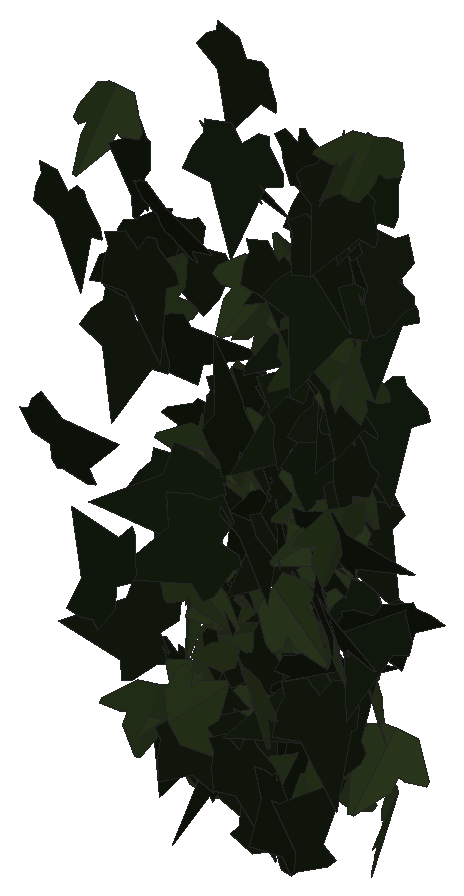
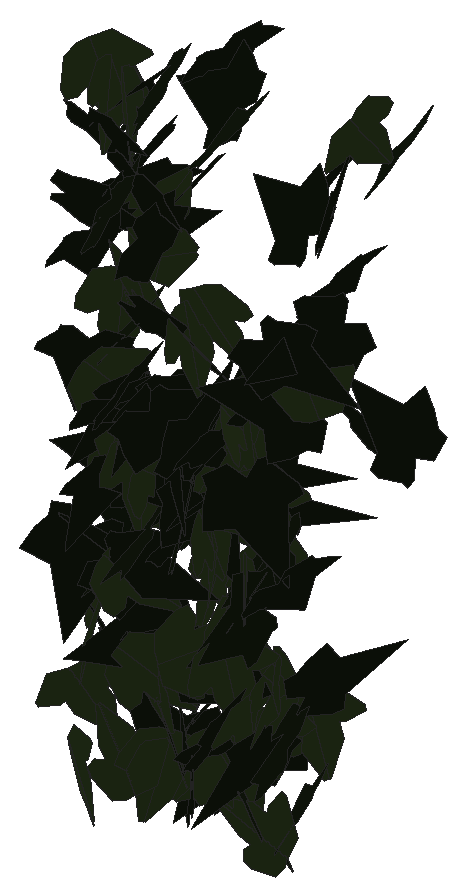
# SketchUp Ruby script. Lengths in inches.
U = 1.inch
M = Sketchup.active_model
def pt(a) = Geom::Point3d.new(a.map { |v| v * U })
def face(e, loops, mat)
  f = e.add_face(loops[0].map { |a| pt(a) })
  loops[1..].each { |l| e.add_face(l.map { |a| pt(a) }).erase! }
  f.material = f.back_material = mat if mat
  f
end
# faces: each face lists its corners as indices into pts; further lists are holes
def faces(e, pts, list, mat = nil) = list.each { |f| face(e, (f[0].is_a?(Array) ? f : [f]).map { |l| l.map { |i| pts[i] } }, mat) }
# xy, xz, yz: faces in a plane at the given z, y or x. An outline is a flat list of corners, or four numbers for a rectangle; further outlines are holes
def ring(l) = l.size == 4 ? [[l[0], l[1]], [l[2], l[1]], [l[2], l[3]], [l[0], l[3]]] : l.each_slice(2).to_a
def flat(e, list, mat, &to3) = list.each { |f| face(e, (f[0].is_a?(Array) ? f : [f]).map { |l| ring(l).map { |u, v| to3.(u, v) } }, mat) }
def xy(e, z, list, mat = nil) = flat(e, list, mat) { |x, y| [x, y, z] }
def xz(e, y, list, mat = nil) = flat(e, list, mat) { |x, z| [x, y, z] }
def yz(e, x, list, mat = nil) = flat(e, list, mat) { |y, z| [x, y, z] }
def lines(e, pts, list) = list.each { |a, b| e.add_line(pt(pts[a]), pt(pts[b])) }
# prism: a flat outline (further loops are holes) pulled along v
def prism(e, loops, v, mat = nil)
  f = face(e, loops, mat); d = Geom::Vector3d.new(v.map { |x| x * U })
  f.pushpull(f.normal.samedirection?(d) ? d.length : -d.length)
end
def box(e, o, s, mat = nil) = prism(e, [[o, [o[0] + s[0], o[1], o[2]], [o[0] + s[0], o[1] + s[1], o[2]], [o[0], o[1] + s[1], o[2]]]], [0, 0, s[2]], mat)
def at(x, y, z, deg = 0) = Geom::Transformation.translation(pt([x, y, z])) * Geom::Transformation.rotation(ORIGIN, Z_AXIS, deg.degrees)
def axes(o, x, y, z) = Geom::Transformation.new([*x, 0, *y, 0, *z, 0, *pt(o).to_a, 1])
def part(name) = M.definitions.add(name)
# library, detail: a bought-in or finely detailed component or shape, given as its bounding box
def library(name, o, s) = part(name).tap { |d| box(d.entities, o, s) }
def detail(e, o, s) = box(e.add_group.entities, o, s)
def put(e, d, t, mat = nil) = e.add_instance(d, t).tap { |i| i.material = mat if mat }
def group(e, t, mat = nil) = e.add_group.tap { |g| g.transformation = t; g.material = mat if mat }.entities
root = M.entities
M.materials.add("efeu1").color = [18, 25, 13]
M.materials.add("efeu2").color = [43, 57, 29]
c1 = part("ivyleaf_9")
p = [[1.54,2.16,1.25],[1.36,2.04,1.19],[-0.21,0.99,0.68],[-0.71,1.11,0.82],[-0.85,0.86,0.67],[-0.8,0.17,0.21],
  [-0.9,-0.01,0.1],[-0.67,-0.16,-0.02],[-0.08,-0.08,-0.05],[-0.03,-0.6,-0.4],[0.65,-0.88,-0.66],[0.83,-0.6,-0.49],
  [1.29,-0.42,-0.43],[1.8125,-0.07,-0.26],[1.21,0.44,0.15]]
faces(c1.entities,p,[[0,1,2,3,4,5,6,7,8,9,10,11,12,13,14]],"efeu1")
c2 = part("ivyleaf_10")
p = [[0,0.5,-0.03],[-0.0625,2.02,-0.43],[-0.19,2.01,-0.46],[-0.54,1.05,-0.29],[-0.52,0.625,-0.18],[-0.83,0.76,-0.28],
  [-1.16,0.64,-0.33],[-1.15,0.33,-0.24],[-0.77,-0.39,0.02],[-0.3,-0.51,0.16],[0.04,-0.48,0.23],[-0.02,2.01,-0.4375],
  [-0.06,2.01,-0.43],[0.04,-0.49,0.23],[0.67,-0.49,0.14],[1.38,0.36,-0.2],[1.375,0.51,-0.24],[0.81,0.65,-0.19],
  [0.62,0.59,-0.15],[0.6,1.09,-0.28],[0.5,1.23,-0.31]]
faces(c2.entities,p,[[0,1,2,3,4,5,6,7,8,9,10],[11,12,0,13,14,15,16,17,18,19,20]],"efeu2")
put(root,c1,axes([31.73,218.72,227.35],[-0.40147,0.0231,-0.29713],[-0.29723,0.00538,0.40202],[0.02177,0.49944,0.00941]))
put(root,c1,axes([30.23,219.64,232.2],[0.13172,-0.45064,0.17197],[0.05266,-0.16376,-0.46948],[0.47945,0.14179,0.00432]))
put(root,c1,axes([31.27,219.81,231.61],[0.13197,-0.48213,-0.01171],[-0.00376,0.01111,-0.49986],[0.48225,0.13202,-0.00069]))
put(root,c1,axes([30.93,220.15,230.29],[-0.06752,-0.47319,0.14675],[0.00171,-0.14833,-0.47749],[0.49542,-0.06397,0.02165]))
put(root,c1,axes([29.68,220.03,228.15],[0.06113,-0.09899,0.48628],[0.39055,-0.29268,-0.10868],[0.30616,0.39312,0.04154]))
put(root,c1,axes([32.48,220.42,233.35],[-0.07704,-0.49374,-0.01691],[-0.00077,0.01723,-0.4997],[0.49403,-0.07697,-0.00341]))
put(root,c1,axes([31.96,220.54,227.23],[-0.34648,-0.16031,0.32288],[-0.26585,-0.18883,-0.37904],[0.24346,-0.43433,0.04562]))
put(root,c2,axes([32.73,220.3125,225.55],[-0.42194,0.26825,0.00295],[-0.00258,0.00144,-0.49999],[-0.26825,-0.42195,0.00017]))
put(root,c2,axes([30.14,220.62,233.11],[0.11451,0.3851,-0.29763],[-0.1191,-0.27429,-0.40073],[-0.47191,0.16267,0.02892]))
put(root,c1,axes([32.77,220.95,223.24],[-0.05974,-0.19541,0.45634],[-0.00949,-0.4591,-0.19784],[0.49633,-0.0323,0.05115]))
put(root,c1,axes([32.27,220.68,224.125],[0.20633,-0.45333,-0.04385],[-0.01284,0.04233,-0.49804],[0.45526,0.20664,0.00583]))
put(root,c2,axes([31.35,220.63,224.4375],[0.31842,-0.09717,-0.37305],[0.35426,-0.11704,0.33287],[-0.15201,-0.4763,-0.00569]))
put(root,c1,axes([31.94,220.82,232.84],[0.24821,-0.25647,0.35016],[0.25958,-0.23557,-0.35654],[0.34786,0.35879,0.01621]))
put(root,c2,axes([33.15,220.98,230.22],[-0.11981,-0.38993,-0.28913],[-0.0887,-0.27521,0.40791],[-0.47726,0.14903,-0.00323]))
put(root,c1,axes([33.51,221,231.3],[-0.26685,-0.42281,0.00461],[0.00267,-0.00713,-0.49994],[0.42283,-0.26679,0.00606]))
put(root,c1,axes([30.71,220.96,231.48],[0.14044,-0.22641,0.4231],[0.30078,-0.30197,-0.26143],[0.37391,0.32795,0.05138]))
put(root,c2,axes([30.75,220.84,224.39],[-0.31553,-0.36661,0.12663],[-0.08358,-0.09514,-0.4837],[0.37876,-0.32641,-0.00125]))
put(root,c2,axes([32.875,220.78,226.55],[0.25402,0.04102,0.42871],[0.42692,0.04159,-0.25693],[-0.05674,0.49658,-0.0139]))
put(root,c1,axes([32.67,220.99,231.42],[0.11716,-0.48258,0.05821],[0.02954,-0.0527,-0.49634],[0.48518,0.11974,0.01617]))
put(root,c2,axes([31.33,220.76,226.52],[-0.38622,-0.04196,-0.31476],[0.31681,-0.01711,-0.38645],[0.02166,-0.49794,0.0398]))
put(root,c1,axes([32.78,220.82,222.875],[-0.16665,-0.04024,0.46969],[0.46722,-0.08038,0.15889],[0.06272,0.49185,0.06439]))
put(root,c1,axes([31.25,221.14,227.27],[-0.33072,0.02226,0.37434],[-0.37126,-0.08976,-0.32266],[0.05284,-0.49137,0.0759]))
put(root,c1,axes([30.1875,221.25,231.76],[-0.107,0.08612,0.48076],[-0.08975,-0.48725,0.06731],[0.4801,-0.07189,0.11973]))
put(root,c1,axes([33.21,221.28,226.37],[-0.05824,-0.02562,0.49593],[0.04701,-0.49738,-0.02017],[0.49437,0.04428,0.06035]))
put(root,c1,axes([33.26,221.1,225.11],[0.03188,-0.48592,-0.11343],[-0.01437,0.11272,-0.48692],[0.49878,0.0343,-0.00678]))
put(root,c1,axes([33.14,221.17,226.38],[0.25511,-0.24553,0.35303],[0.24593,-0.25343,-0.35397],[0.35276,0.35425,-0.00854]))
put(root,c1,axes([33.48,221.38,232.59],[-0.1259,-0.42386,0.23344],[0.01442,-0.24439,-0.43596],[0.48367,-0.10304,0.07376]))
put(root,c1,axes([30.3,221.38,224.96],[-0.13614,-0.05369,0.4781],[-0.37081,-0.30488,-0.13982],[0.30654,-0.39264,0.0432]))
put(root,c2,axes([33.5,221.21,227.8125],[-0.07464,-0.4874,0.08288],[0.00211,-0.08413,-0.49287],[0.49439,-0.07322,0.01461]))
put(root,c1,axes([31.93,221.04,228.45],[-0.07383,-0.37451,0.32294],[0.06665,0.316,0.38171],[-0.49001,0.09941,0.00326]))
put(root,c1,axes([31.86,221.43,227.14],[0.11738,-0.41649,0.25051],[0.10856,-0.22874,-0.43115],[0.47375,0.15561,0.03673]))
put(root,c1,axes([33.16,221.25,231.95],[0.18219,-0.45437,-0.10175],[-0.03884,0.09405,-0.48954],[0.464,0.18629,-0.00103]))
put(root,c2,axes([30.88,221.55,224.22],[-0.04596,-0.16134,0.47102],[-0.01392,-0.47242,-0.16318],[0.49769,-0.02811,0.03893]))
put(root,c2,axes([33.11,221.41,226.11],[0.10408,-0.14756,0.46625],[0.43462,-0.19065,-0.15735],[0.22422,0.43804,0.08858]))
put(root,c1,axes([32.79,221.28,233.08],[0.31104,-0.39005,-0.03339],[-0.01848,0.02797,-0.49888],[0.39104,0.31158,0.00298]))
put(root,c2,axes([33,221.34,230.95],[-0.42991,0.00075,-0.25529],[-0.25496,-0.02691,0.42927],[-0.01309,0.49927,0.02353]))
put(root,c2,axes([33.51,221.36,230.33],[0.41534,-0.2782,0.00988],[0.00882,-0.00458,-0.4999],[0.27824,0.41543,0.0011]))
put(root,c1,axes([31.21,221.22,223.9375],[-0.06721,-0.32468,-0.37426],[0.06289,0.36904,-0.33144],[0.49145,-0.09163,-0.00877]))
put(root,c1,axes([33.1,221.27,227.37],[0.30427,-0.10914,0.38145],[0.36377,-0.11517,-0.32312],[0.1584,0.47416,0.00932]))
put(root,c1,axes([33,221.63,224.74],[-0.35677,-0.15229,0.31547],[-0.26316,-0.18067,-0.38484],[0.23121,-0.44064,0.04876]))
put(root,c1,axes([30.79,221.29,226.88],[0.43551,-0.24409,-0.02739],[-0.01944,0.02134,-0.49917],[0.24486,0.43585,0.00909]))
put(root,c2,axes([33.24,221.54,227.51],[0.20989,0.16261,-0.42368],[-0.35789,-0.22772,-0.26469],[-0.27904,0.41437,0.0208]))
put(root,c2,axes([31.62,221.21,228.33],[-0.30317,0.10915,0.38233],[-0.37409,0.08457,-0.32079],[-0.1347,-0.48055,0.03039]))
put(root,c2,axes([33.74,221.52,233.28],[-0.29217,-0.36755,0.17189],[-0.06653,-0.16555,-0.46708],[0.40027,-0.2958,0.04783]))
put(root,c1,axes([33.14,221.77,229.42],[-0.02328,-0.40036,0.29861],[0.10503,-0.29618,-0.38891],[0.48829,0.04463,0.09789]))
put(root,c2,axes([31.35,221.7,228.875],[0.161,-0.33734,0.33208],[0.15744,-0.29263,-0.3736],[0.44642,0.22486,0.012]))
put(root,c2,axes([33.45,221.38,229.89],[-0.48414,-0.12229,0.0255],[-0.02433,-0.0078,-0.49935],[0.12253,-0.48475,0.0016]))
put(root,c1,axes([31.14,221.75,226.18],[0.0984,-0.38481,0.30371],[0.10075,-0.28728,-0.39664],[0.47976,0.13926,0.021]))
put(root,c1,axes([33.32,221.3125,224.2],[-0.28497,0.35014,0.21493],[0.13569,-0.16668,0.45145],[0.38779,0.31563,-0.00002]))
put(root,c1,axes([32.2,221.88,226.83],[-0.1631,-0.33248,0.33594],[-0.13216,-0.30912,-0.3701],[0.4538,-0.20952,0.01295]))
put(root,c2,axes([31.51,221.4375,228.4375],[-0.44715,-0.09587,-0.20215],[0.20362,0.01281,-0.45648],[0.09271,-0.49056,0.02758]))
put(root,c1,axes([30.21,221.86,223.27],[0.02299,-0.35402,0.35233],[0.05023,-0.34928,-0.35423],[0.49694,0.05168,0.0195]))
put(root,c1,axes([32.02,221.54,227.46],[-0.06162,0.38893,-0.30812],[0.05705,-0.30287,-0.39372],[-0.4929,-0.08368,-0.00705]))
put(root,c1,axes([31.22,221.61,223.38],[-0.40293,0.194,-0.22362],[0.20317,-0.09349,-0.44719],[-0.21532,-0.45125,-0.0035]))
put(root,c2,axes([33.1,221.74,228.16],[-0.25038,-0.24771,0.3549],[-0.1855,-0.30902,-0.34655],[0.39103,-0.3052,0.06284]))
put(root,c2,axes([33.26,221.46,232.96],[0.18677,-0.43761,-0.15368],[-0.0279,0.15477,-0.47462],[0.46297,0.18587,0.0334]))
put(root,c1,axes([32.64,221.95,231.15],[0.02089,-0.21706,-0.44994],[0.17586,-0.41832,0.20997],[-0.46759,-0.16702,0.05886]))
put(root,c2,axes([31.54,221.67,224.96],[-0.32017,-0.37486,-0.08349],[-0.04398,-0.07219,0.4928],[-0.38152,0.32291,0.01325]))
put(root,c2,axes([33.52,221.45,233.05],[-0.02878,-0.46335,-0.1857],[0.01239,0.18528,-0.46424],[0.49902,-0.03132,0.00082]))
put(root,c1,axes([33.72,221.73,226.3],[-0.41573,-0.15907,-0.22774],[0.22161,0.05725,-0.44453],[0.1675,-0.47055,0.0229]))
put(root,c1,axes([32.57,221.92,228.82],[-0.3457,-0.28285,0.2247],[-0.15714,-0.16229,-0.44606],[0.32527,-0.37902,0.02331]))
put(root,c2,axes([32.5625,221.93,227.69],[-0.09493,-0.29025,0.39591],[0.1702,-0.39769,-0.25074],[0.46046,0.08716,0.17431]))
put(root,c1,axes([33.42,221.5,228.08],[-0.10711,0.0721,0.48304],[-0.3727,0.30752,-0.12854],[-0.31563,-0.3876,-0.01214]))
put(root,c2,axes([32.91,221.625,227.71],[-0.30263,-0.39788,-0.01034],[0.00663,0.00795,-0.49989],[0.39796,-0.3027,0.00046]))
put(root,c1,axes([32.375,221.78,223.99],[-0.33485,0.09349,-0.35936],[0.35062,-0.07971,-0.34744],[-0.12225,-0.48467,-0.01218]))
put(root,c2,axes([30.98,221.65,227.88],[-0.40867,-0.24216,0.15605],[-0.14259,-0.0653,-0.47477],[0.25032,-0.43254,-0.01569]))
put(root,c2,axes([30.91,221.62,227.69],[-0.27014,-0.11013,-0.40607],[0.42003,-0.04257,-0.26789],[0.02444,-0.48586,0.11552]))
put(root,c1,axes([30.32,221.46,229.27],[0.20473,0.20979,-0.40506],[0.27889,0.29378,0.29311],[0.36098,-0.34595,0.00328]))
put(root,c1,axes([33.93,221.79,231.27],[-0.43147,0.02346,0.25156],[-0.25153,0.00692,-0.43207],[-0.02375,-0.4994,0.00583]))
put(root,c1,axes([32.14,221.55,227.61],[0.12959,-0.01067,-0.4828],[0.34252,0.35441,0.0841],[0.34042,-0.35254,0.09917]))
put(root,c1,axes([29.85,221.32,230.56],[0.03654,0.07557,-0.4929],[-0.03158,0.49358,0.07333],[0.49766,0.02577,0.04084]))
put(root,c1,axes([31.36,221.62,225.14],[-0.03974,-0.01724,-0.49812],[0.37739,0.32537,-0.04137],[0.32557,-0.37926,-0.01285]))
put(root,c1,axes([33.5,221.9,232.61],[-0.46274,-0.09896,-0.16149],[0.16167,0.01569,-0.47288],[0.09866,-0.48986,0.01748]))
put(root,c1,axes([33.5,221.92,230.95],[-0.04543,-0.49433,-0.05981],[-0.00017,0.06007,-0.49638],[0.49793,-0.04508,-0.00563]))
put(root,c2,axes([31.7,221.77,230.46],[0.44234,-0.02533,-0.23171],[-0.23118,0.0158,-0.44306],[0.02977,0.49911,0.00227]))
put(root,c1,axes([30.28,222.03,226.89],[-0.11208,-0.48332,0.06195],[-0.01455,-0.06022,-0.49615],[0.48706,-0.11302,-0.00056]))
put(root,c2,axes([31.48,221.95,226.92],[-0.21619,0.24377,-0.37926],[0.16313,-0.34981,-0.31784],[-0.4203,-0.26116,0.07171]))
put(root,c2,axes([29.95,221.75,229.61],[-0.41539,-0.16535,0.22386],[0.2082,0.08228,0.44708],[-0.18469,0.46464,0.0005]))
put(root,c1,axes([32.58,221.41,225.1],[0.31811,0.14978,0.35549],[0.28819,0.21401,-0.34806],[-0.25642,0.42634,0.04983]))
put(root,c2,axes([33.29,222.03,228.95],[-0.24961,-0.23668,0.36287],[-0.10688,-0.37221,-0.31629],[0.41985,-0.23546,0.13523]))
put(root,c1,axes([32.72,221.93,232.03],[-0.33999,-0.11732,-0.34733],[0.35315,0.02239,-0.35325],[0.09844,-0.48552,0.06764]))
put(root,c1,axes([31.88,222.06,227.2],[0.15045,-0.13223,-0.45812],[0.42158,-0.18756,0.19259],[-0.22279,-0.44422,0.05506]))
put(root,c2,axes([32.96,222.01,226.18],[-0.20757,-0.22122,0.39747],[-0.18813,-0.35603,-0.2964],[0.41415,-0.27259,0.06457]))
put(root,c1,axes([31.39,221.875,228.7],[0.08153,-0.47938,-0.11641],[-0.01028,0.11631,-0.48618],[0.4932,0.08166,0.00911]))
put(root,c1,axes([32.95,221.52,228.62],[0.09158,-0.18517,-0.45533],[-0.05404,0.45656,-0.19654],[0.48856,0.08521,0.06361]))
put(root,c2,axes([31.33,221.91,223.88],[-0.2558,-0.35512,0.24178],[-0.14673,-0.19225,-0.43762],[0.40378,-0.29484,-0.00585]))
put(root,c1,axes([30.32,221.88,224.35],[0.33058,-0.3629,0.09498],[0.0602,-0.07363,-0.49087],[0.37026,0.33598,-0.00499]))
put(root,c2,axes([31.97,222.09,225.25],[-0.12855,0.0007,-0.48319],[-0.32613,-0.36906,0.08623],[-0.35653,0.33733,0.09534]))
put(root,c1,axes([33.02,222.02,226.28],[-0.08182,-0.02986,-0.49236],[-0.20035,-0.45405,0.06083],[-0.45074,0.20724,0.06233]))
put(root,c2,axes([32.42,221.73,223.56],[-0.40331,-0.27259,-0.11416],[0.09986,0.05609,-0.48671],[0.27815,-0.41539,0.00919]))
put(root,c2,axes([31.51,222,227.3],[0.04003,-0.4499,0.21444],[0.12309,-0.19954,-0.44163],[0.48296,0.08815,0.09478]))
put(root,c2,axes([33.72,221.9,224.23],[0.37311,0.26342,-0.20346],[-0.16111,-0.12451,-0.45666],[-0.29126,0.40633,-0.00804]))
put(root,c2,axes([31.92,221.86,230.13],[-0.05362,-0.49694,0.01311],[0.00015,-0.01321,-0.49983],[0.49712,-0.0536,0.00157]))
put(root,c2,axes([32.77,221.74,224.76],[0.33826,-0.1768,-0.32298],[-0.25525,0.20351,-0.37872],[0.26537,0.4211,0.04742]))
put(root,c2,axes([30.9,221.91,224.83],[0.02462,0.47185,-0.16355],[-0.0203,-0.16267,-0.47236],[-0.49898,0.0299,0.01115]))
put(root,c2,axes([31.09,221.68,226.58],[0.17145,-0.35916,-0.30267],[-0.07908,0.29553,-0.39548],[0.46298,0.18348,0.04454]))
put(root,c2,axes([31.24,221.98,225.4375],[-0.28355,-0.39553,0.11471],[0.02344,-0.15455,-0.47494],[0.41116,-0.26396,0.10619]))
put(root,c2,axes([33.09,221.8,228.27],[-0.47485,0.04885,-0.14875],[0.149,-0.00491,-0.47726],[-0.04809,-0.49758,-0.00989]))
put(root,c1,axes([32.48,221.78,228.88],[0.12143,-0.36015,-0.32488],[-0.11036,0.30561,-0.38003],[0.47231,0.164,-0.00528]))
put(root,c1,axes([33.74,221.65,226.27],[0.294,0.38822,-0.11335],[-0.07582,-0.08474,-0.4869],[-0.39726,0.30349,0.00904]))
put(root,c1,axes([31.28,221.78,224],[0.0112,-0.3243,-0.3804],[0.04035,0.37984,-0.32264],[0.49824,-0.02347,0.03467]))
put(root,c2,axes([32.71,222.04,224.89],[-0.23356,-0.12616,0.42371],[-0.32417,-0.27696,-0.26116],[0.3006,-0.39671,0.04758]))
put(root,c1,axes([31.71,222.125,223.22],[-0.01399,0.07892,0.49353],[0.09732,-0.48385,0.08013],[0.49024,0.0983,-0.00183]))
put(root,c1,axes([32.97,222.12,228.72],[-0.16718,-0.46953,-0.03993],[0.01466,0.03717,-0.4984],[0.471,-0.16781,0.00134]))
put(root,c2,axes([33.56,221.76,225.23],[-0.28622,0.40018,0.08909],[-0.06367,0.06395,-0.49179],[-0.405,-0.29286,0.01435]))
put(root,c1,axes([33.49,221.97,229.33],[-0.24228,-0.31896,-0.29927],[0.17005,0.24651,-0.40039],[0.40297,-0.2958,-0.01097]))
put(root,c2,axes([31.3,221.71,223.96],[-0.24911,-0.23746,-0.3627],[0.29123,0.21821,-0.34288],[0.32113,-0.3821,0.0296]))
put(root,c1,axes([32.3,222.13,228.74],[0.02695,0.06994,-0.49435],[-0.11898,-0.47991,-0.07439],[-0.48489,0.12164,-0.00923]))
put(root,c1,axes([30.46,222.07,230.4],[0.00571,-0.00663,-0.49992],[-0.30117,-0.39912,0.00185],[-0.39908,0.3011,-0.00855]))
put(root,c1,axes([30.94,221.87,228.1],[0.16542,0.2568,-0.39584],[-0.28142,-0.283,-0.30119],[-0.37874,0.32244,0.05091]))
put(root,c1,axes([33.22,221.84,227.5],[0.05544,-0.3688,-0.33303],[-0.06047,0.3276,-0.37286],[0.49322,0.08162,-0.00828]))
put(root,c1,axes([31.78,222.15,228.26],[-0.00582,0.18203,0.46565],[-0.29306,-0.37853,0.14431],[0.40507,-0.27125,0.1111]))
put(root,c1,axes([32.54,222.07,230.16],[-0.49537,0.01621,0.06592],[-0.06618,-0.00703,-0.49555],[-0.01514,-0.49969,0.00911]))
put(root,c1,axes([31.03,222.3125,233.3],[-0.04969,-0.40582,0.28783],[0.08626,-0.2919,-0.39668],[0.48999,0.01023,0.09902]))
put(root,c1,axes([32.92,222.27,231.51],[0.09553,-0.37914,0.31165],[0.09129,-0.29823,-0.3908],[0.48222,0.13156,0.01225]))
put(root,c1,axes([32.74,222.33,228.96],[-0.0398,-0.41034,0.2829],[-0.03044,-0.28127,-0.41226],[0.49748,-0.05004,-0.00259]))
put(root,c1,axes([32.59,221.9,226.82],[0.38839,-0.29206,-0.11771],[-0.06336,0.1106,-0.48348],[0.30845,0.39047,0.0489]))
put(root,c2,axes([30.4375,221.9375,222.91],[-0.18037,-0.06589,0.46166],[0.45132,0.09994,0.19059],[-0.11739,0.48546,0.02342]))
put(root,c2,axes([33.63,222.06,223.2],[0.26369,-0.4244,0.01879],[0.00856,-0.0168,-0.49964],[0.42473,0.26382,-0.00159]))
put(root,c1,axes([32.32,221.78,228.24],[0.04123,0.04394,-0.49636],[-0.49472,0.0632,-0.0355],[0.05962,0.49404,0.04869]))
put(root,c1,axes([31.22,222.42,224.35],[-0.09842,-0.30637,0.38269],[-0.10218,-0.36893,-0.32163],[0.47945,-0.14151,0.01001]))
put(root,c2,axes([30.29,222.21,225.3125],[-0.08124,0.35408,-0.34355],[0.08047,-0.33401,-0.36327],[-0.48675,-0.11432,-0.00272]))
put(root,c1,axes([30.625,221.98,226.34],[0.47245,-0.16191,0.024],[0.02277,-0.00758,-0.49942],[0.16209,0.473,0.00021]))
put(root,c2,axes([32.71,222.1,223.21],[-0.3902,-0.14936,0.27465],[0.28513,0.01016,0.41061],[-0.12824,0.47706,0.07725]))
put(root,c1,axes([30.67,221.79,224.26],[0.15699,-0.15565,-0.44847],[-0.14148,0.43555,-0.2007],[0.45314,0.18992,0.09271]))
